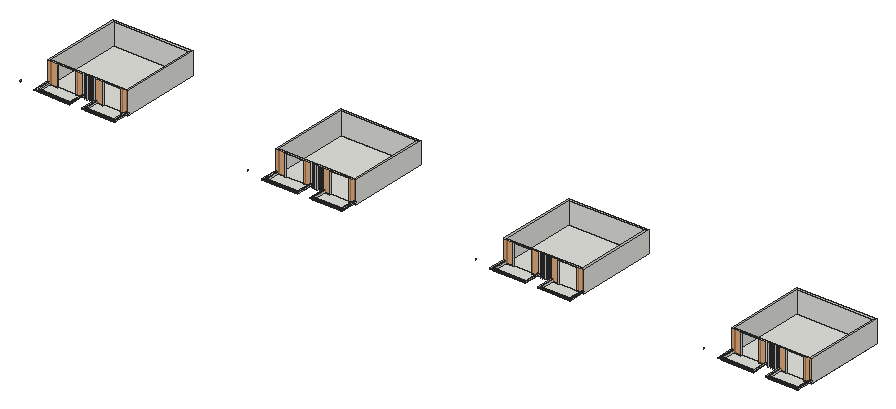
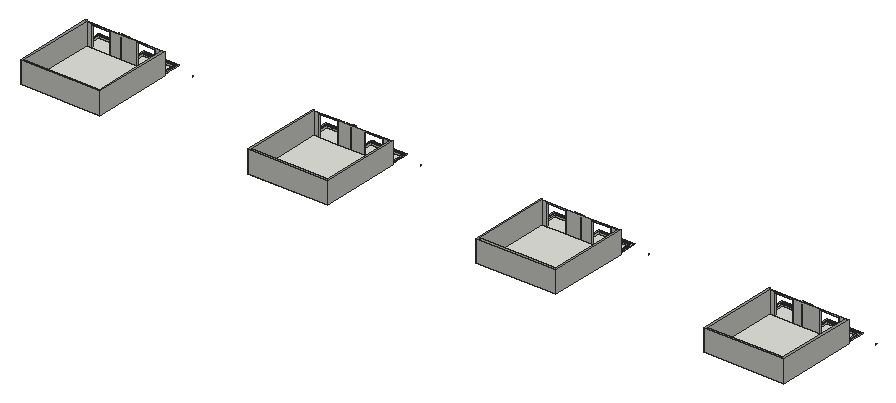
# SketchUp Ruby script. Lengths in inches.
U = 1.inch
M = Sketchup.active_model
def pt(a) = Geom::Point3d.new(a.map { |v| v * U })
def face(e, loops, mat)
  f = e.add_face(loops[0].map { |a| pt(a) })
  loops[1..].each { |l| e.add_face(l.map { |a| pt(a) }).erase! }
  f.material = f.back_material = mat if mat
  f
end
# faces: each face lists its corners as indices into pts; further lists are holes
def faces(e, pts, list, mat = nil) = list.each { |f| face(e, (f[0].is_a?(Array) ? f : [f]).map { |l| l.map { |i| pts[i] } }, mat) }
# xy, xz, yz: faces in a plane at the given z, y or x. An outline is a flat list of corners, or four numbers for a rectangle; further outlines are holes
def ring(l) = l.size == 4 ? [[l[0], l[1]], [l[2], l[1]], [l[2], l[3]], [l[0], l[3]]] : l.each_slice(2).to_a
def flat(e, list, mat, &to3) = list.each { |f| face(e, (f[0].is_a?(Array) ? f : [f]).map { |l| ring(l).map { |u, v| to3.(u, v) } }, mat) }
def xy(e, z, list, mat = nil) = flat(e, list, mat) { |x, y| [x, y, z] }
def xz(e, y, list, mat = nil) = flat(e, list, mat) { |x, z| [x, y, z] }
def yz(e, x, list, mat = nil) = flat(e, list, mat) { |y, z| [x, y, z] }
def lines(e, pts, list) = list.each { |a, b| e.add_line(pt(pts[a]), pt(pts[b])) }
# prism: a flat outline (further loops are holes) pulled along v
def prism(e, loops, v, mat = nil)
  f = face(e, loops, mat); d = Geom::Vector3d.new(v.map { |x| x * U })
  f.pushpull(f.normal.samedirection?(d) ? d.length : -d.length)
end
def box(e, o, s, mat = nil) = prism(e, [[o, [o[0] + s[0], o[1], o[2]], [o[0] + s[0], o[1] + s[1], o[2]], [o[0], o[1] + s[1], o[2]]]], [0, 0, s[2]], mat)
def at(x, y, z, deg = 0) = Geom::Transformation.translation(pt([x, y, z])) * Geom::Transformation.rotation(ORIGIN, Z_AXIS, deg.degrees)
def axes(o, x, y, z) = Geom::Transformation.new([*x, 0, *y, 0, *z, 0, *pt(o).to_a, 1])
def part(name) = M.definitions.add(name)
# library, detail: a bought-in or finely detailed component or shape, given as its bounding box
def library(name, o, s) = part(name).tap { |d| box(d.entities, o, s) }
def detail(e, o, s) = box(e.add_group.entities, o, s)
def put(e, d, t, mat = nil) = e.add_instance(d, t).tap { |i| i.material = mat if mat }
def group(e, t, mat = nil) = e.add_group.tap { |g| g.transformation = t; g.material = mat if mat }.entities
root = M.entities
M.materials.add("[0043_SaddleBrown]4").color = [124, 123, 122]
M.materials.add("[Granite Light Gray]").color = [149, 148, 144]
M.materials.add("[Wood Floor]").color = [224, 152, 88]
M.materials["[Wood Floor]"].alpha = 0.68
xy(root,652.4375,[[563.08,570.83,736.65,570.83,736.65,651.03,703.26,651.03,703.26,657.03,602.01,657.03,602.01,651.03,563.08,651.03],[820.97,570.83,978.86,570.83,978.86,651.03,951.01,651.03,951.01,657.03,849.76,657.03,849.76,651.03,820.97,651.03],[1813.71,570.83,1987.28,570.83,1987.28,651.03,1953.89,651.03,1953.89,657.03,1852.64,657.03,1852.64,651.03,1813.71,651.03],[2071.59,570.83,2229.49,570.83,2229.49,651.03,2201.63,651.03,2201.63,657.03,2100.38,657.03,2100.38,651.03,2071.59,651.03],[3064.33,570.83,3237.9,570.83,3237.9,651.03,3204.51,651.03,3204.51,657.03,3103.26,657.03,3103.26,651.03,3064.33,651.03],
  [3322.22,570.83,3480.11,570.83,3480.11,651.03,3452.26,651.03,3452.26,657.03,3351.01,657.03,3351.01,651.03,3322.22,651.03],[4314.96,570.83,4488.53,570.83,4488.53,651.03,4455.14,651.03,4455.14,657.03,4353.89,657.03,4353.89,651.03,4314.96,651.03],[4572.84,570.83,4730.74,570.83,4730.74,651.03,4702.88,651.03,4702.88,657.03,4601.63,657.03,4601.63,651.03,4572.84,651.03],[551.76,651.03,551.76,1096.5,990.19,1096.5,990.19,651.03,951.01,651.03,951.01,657.03,978.86,657.03,978.86,1085.17,563.08,1085.17,563.08,657.03,602.01,657.03,602.01,651.03],[1802.38,651.03,1802.38,1096.5,2240.81,1096.5,2240.81,651.03,2201.63,651.03,2201.63,657.03,2229.49,657.03,2229.49,1085.17,1813.71,1085.17,1813.71,657.03,1852.64,657.03,1852.64,651.03],
  [3053.01,651.03,3053.01,1096.5,3491.44,1096.5,3491.44,651.03,3452.26,651.03,3452.26,657.03,3480.11,657.03,3480.11,1085.17,3064.33,1085.17,3064.33,657.03,3103.26,657.03,3103.26,651.03],[4303.63,651.03,4303.63,1096.5,4742.06,1096.5,4742.06,651.03,4702.88,651.03,4702.88,657.03,4730.74,657.03,4730.74,1085.17,4314.96,1085.17,4314.96,657.03,4353.89,657.03,4353.89,651.03],[563.08,657.03,978.86,1085.17],[1813.71,657.03,2229.49,1085.17],[3064.33,657.03,3480.11,1085.17],
  [4314.96,657.03,4730.74,1085.17]])
xy(root,662.4375,[[549.88,558.125,744.19,559.875],[812.81,558.125,990.19,559.875],[990.19,558.125,991.94,651.03],[1800.51,558.125,1994.82,559.875],[2063.43,558.125,2240.81,559.875],
  [2240.81,558.125,2242.56,651.03],[3051.13,558.125,3245.44,559.875],[3314.06,558.125,3491.44,559.875],[3491.44,558.125,3493.19,651.03],[4301.76,558.125,4496.07,559.875],
  [4564.68,558.125,4742.06,559.875],[4742.06,558.125,4743.81,651.03],[549.88,559.875,551.76,640.11],[551.76,559.875,551.76,651.03,563.08,651.03,563.08,570.83,736.65,570.83,736.65,651.03,742.44,651.03,742.44,559.875],[742.44,559.875,744.19,647.91],
  [812.81,559.875,812.81,648.85,814.68,648.85,814.68,651.03,814.89,651.03,814.89,559.875],[814.89,559.875,814.89,651.03,820.97,651.03,820.97,570.83,978.86,570.83,978.86,651.03,990.19,651.03,990.19,559.875],[1800.51,559.875,1802.38,640.11],[1802.38,559.875,1802.38,651.03,1813.71,651.03,1813.71,570.83,1987.28,570.83,1987.28,651.03,1993.07,651.03,1993.07,559.875],[1993.07,559.875,1994.82,647.91],
  [2063.43,559.875,2063.43,648.85,2065.31,648.85,2065.31,651.03,2065.52,651.03,2065.52,559.875],[2065.52,559.875,2065.52,651.03,2071.59,651.03,2071.59,570.83,2229.49,570.83,2229.49,651.03,2240.81,651.03,2240.81,559.875],[3051.13,559.875,3053.01,640.11],[3053.01,559.875,3053.01,651.03,3064.33,651.03,3064.33,570.83,3237.9,570.83,3237.9,651.03,3243.69,651.03,3243.69,559.875],[3243.69,559.875,3245.44,647.91],
  [3314.06,559.875,3314.06,648.85,3315.93,648.85,3315.93,651.03,3316.14,651.03,3316.14,559.875],[3316.14,559.875,3316.14,651.03,3322.22,651.03,3322.22,570.83,3480.11,570.83,3480.11,651.03,3491.44,651.03,3491.44,559.875],[4301.76,559.875,4303.63,640.11],[4303.63,559.875,4303.63,651.03,4314.96,651.03,4314.96,570.83,4488.53,570.83,4488.53,651.03,4494.32,651.03,4494.32,559.875],[4494.32,559.875,4496.07,647.91],
  [4564.68,559.875,4564.68,648.85,4566.56,648.85,4566.56,651.03,4566.77,651.03,4566.77,559.875],[4566.77,559.875,4566.77,651.03,4572.84,651.03,4572.84,570.83,4730.74,570.83,4730.74,651.03,4742.06,651.03,4742.06,559.875]])
xz(root,558.125,[[549.88,662.4375,744.19,665.9375],[812.81,662.4375,991.94,665.9375],[1800.51,662.4375,1994.82,665.9375],[2063.43,662.4375,2242.56,665.9375],[3051.13,662.4375,3245.44,665.9375],
  [3314.06,662.4375,3493.19,665.9375],[4301.76,662.4375,4496.07,665.9375],[4564.68,662.4375,4743.81,665.9375]],"[Granite Light Gray]")
xz(root,570.83,[[563.08,652.4375,736.65,662.4375],[820.97,652.4375,978.86,662.4375],[1813.71,652.4375,1987.28,662.4375],[2071.59,652.4375,2229.49,662.4375],[3064.33,652.4375,3237.9,662.4375],
  [3322.22,652.4375,3480.11,662.4375],[4314.96,652.4375,4488.53,662.4375],[4572.84,652.4375,4730.74,662.4375],[563.08,662.4375,736.65,665.9375],[820.97,662.4375,978.86,665.9375],
  [1813.71,662.4375,1987.28,665.9375],[2071.59,662.4375,2229.49,665.9375],[3064.33,662.4375,3237.9,665.9375],[3322.22,662.4375,3480.11,665.9375],[4314.96,662.4375,4488.53,665.9375],
  [4572.84,662.4375,4730.74,665.9375]])
xz(root,589.17,[[449.07,657.09,449.07,663.29,448.85,662.79,448.66,662.27,448.52,661.76,448.42,661.24,448.35,660.72,448.33,660.19,448.35,659.67,448.42,659.14,448.52,658.625,448.66,658.11,448.85,657.6],[1699.7,657.09,1699.7,663.29,1699.47,662.79,1699.29,662.27,1699.14,661.76,1699.04,661.24,1698.98,660.72,1698.96,660.19,1698.98,659.67,1699.04,659.14,1699.14,658.625,1699.29,658.11,1699.47,657.6],[2950.32,657.09,2950.32,663.29,2950.1,662.79,2949.91,662.27,2949.77,661.76,2949.67,661.24,2949.6,660.72,2949.58,660.19,2949.6,659.67,2949.67,659.14,2949.77,658.625,2949.91,658.11,2950.1,657.6],[4200.95,657.09,4200.95,663.29,4200.72,662.79,4200.54,662.27,4200.39,661.76,4200.29,661.24,4200.23,660.72,4200.21,660.19,4200.23,659.67,4200.29,659.14,4200.39,658.625,4200.54,658.11,4200.72,657.6]],"[0043_SaddleBrown]4")
xz(root,640.11,[[549.88,662.4375,551.76,665.9375],[1800.51,662.4375,1802.38,665.9375],[3051.13,662.4375,3053.01,665.9375],[4301.76,662.4375,4303.63,665.9375]])
xz(root,647.91,[[742.44,662.4375,744.19,665.9375],[1993.07,662.4375,1994.82,665.9375],[3243.69,662.4375,3245.44,665.9375],[4494.32,662.4375,4496.07,665.9375]])
xz(root,648.85,[[812.81,662.4375,814.68,665.9375],[2063.43,662.4375,2065.31,665.9375],[3314.06,662.4375,3315.93,665.9375],[4564.68,662.4375,4566.56,665.9375]])
xz(root,651.03,[[551.76,652.4375,563.08,662.4375],[978.86,652.4375,990.19,662.4375],[1802.38,652.4375,1813.71,662.4375],[2229.49,652.4375,2240.81,662.4375],[3053.01,652.4375,3064.33,662.4375],
  [3480.11,652.4375,3491.44,662.4375],[4303.63,652.4375,4314.96,662.4375],[4730.74,652.4375,4742.06,662.4375],[551.76,662.4375,563.08,665.9375],[736.65,662.4375,742.44,665.9375],
  [814.68,662.4375,820.97,665.9375],[978.86,662.4375,990.19,665.9375],[990.19,662.4375,991.94,665.9375],[1802.38,662.4375,1813.71,665.9375],[1987.28,662.4375,1993.07,665.9375],
  [2065.31,662.4375,2071.59,665.9375],[2229.49,662.4375,2240.81,665.9375],[2240.81,662.4375,2242.56,665.9375],[3053.01,662.4375,3064.33,665.9375],[3237.9,662.4375,3243.69,665.9375],
  [3315.93,662.4375,3322.22,665.9375],[3480.11,662.4375,3491.44,665.9375],[3491.44,662.4375,3493.19,665.9375],[4303.63,662.4375,4314.96,665.9375],[4488.53,662.4375,4494.32,665.9375],
  [4566.56,662.4375,4572.84,665.9375],[4730.74,662.4375,4742.06,665.9375],[4742.06,662.4375,4743.81,665.9375]])
xz(root,651.03,[[563.08,652.4375,602.01,652.4375,602.01,766.875,703.26,766.875,703.26,652.4375,736.65,652.4375,736.65,665.9375,742.44,665.9375,742.44,771.4375,551.76,771.4375,551.76,665.9375,563.08,665.9375],[820.97,652.4375,849.76,652.4375,849.76,766.875,951.01,766.875,951.01,652.4375,978.86,652.4375,978.86,665.9375,990.19,665.9375,990.19,772.4375,978.86,772.4375,978.86,776.0625,977.59,776.0625,977.59,771.4375,814.89,771.4375,814.89,665.9375,820.97,665.9375],[1813.71,652.4375,1852.64,652.4375,1852.64,766.875,1953.89,766.875,1953.89,652.4375,1987.28,652.4375,1987.28,665.9375,1993.07,665.9375,1993.07,771.4375,1802.38,771.4375,1802.38,665.9375,1813.71,665.9375],[2071.59,652.4375,2100.38,652.4375,2100.38,766.875,2201.63,766.875,2201.63,652.4375,2229.49,652.4375,2229.49,665.9375,2240.81,665.9375,2240.81,772.4375,2229.49,772.4375,2229.49,776.0625,2228.22,776.0625,2228.22,771.4375,2065.52,771.4375,2065.52,665.9375,2071.59,665.9375],[3064.33,652.4375,3103.26,652.4375,3103.26,766.875,3204.51,766.875,3204.51,652.4375,3237.9,652.4375,3237.9,665.9375,3243.69,665.9375,3243.69,771.4375,3053.01,771.4375,3053.01,665.9375,3064.33,665.9375],
  [3322.22,652.4375,3351.01,652.4375,3351.01,766.875,3452.26,766.875,3452.26,652.4375,3480.11,652.4375,3480.11,665.9375,3491.44,665.9375,3491.44,772.4375,3480.11,772.4375,3480.11,776.0625,3478.84,776.0625,3478.84,771.4375,3316.14,771.4375,3316.14,665.9375,3322.22,665.9375],[4314.96,652.4375,4353.89,652.4375,4353.89,766.875,4455.14,766.875,4455.14,652.4375,4488.53,652.4375,4488.53,665.9375,4494.32,665.9375,4494.32,771.4375,4303.63,771.4375,4303.63,665.9375,4314.96,665.9375],[4572.84,652.4375,4601.63,652.4375,4601.63,766.875,4702.88,766.875,4702.88,652.4375,4730.74,652.4375,4730.74,665.9375,4742.06,665.9375,4742.06,772.4375,4730.74,772.4375,4730.74,776.0625,4729.47,776.0625,4729.47,771.4375,4566.77,771.4375,4566.77,665.9375,4572.84,665.9375]],"[Wood Floor]")
xz(root,657.03,[[563.08,652.4375,563.08,772.4375,978.86,772.4375,978.86,652.4375,951.01,652.4375,951.01,766.875,849.76,766.875,849.76,652.4375,703.26,652.4375,703.26,766.875,602.01,766.875,602.01,652.4375],[1813.71,652.4375,1813.71,772.4375,2229.49,772.4375,2229.49,652.4375,2201.63,652.4375,2201.63,766.875,2100.38,766.875,2100.38,652.4375,1953.89,652.4375,1953.89,766.875,1852.64,766.875,1852.64,652.4375],[3064.33,652.4375,3064.33,772.4375,3480.11,772.4375,3480.11,652.4375,3452.26,652.4375,3452.26,766.875,3351.01,766.875,3351.01,652.4375,3204.51,652.4375,3204.51,766.875,3103.26,766.875,3103.26,652.4375],[4314.96,652.4375,4314.96,772.4375,4730.74,772.4375,4730.74,652.4375,4702.88,652.4375,4702.88,766.875,4601.63,766.875,4601.63,652.4375,4455.14,652.4375,4455.14,766.875,4353.89,766.875,4353.89,652.4375]])
xz(root,1085.17,[[563.08,652.4375,978.86,772.4375],[1813.71,652.4375,2229.49,772.4375],[3064.33,652.4375,3480.11,772.4375],[4314.96,652.4375,4730.74,772.4375]])
xz(root,1096.5,[[551.76,652.4375,990.19,772.4375],[1802.38,652.4375,2240.81,772.4375],[3053.01,652.4375,3491.44,772.4375],[4303.63,652.4375,4742.06,772.4375]])
yz(root,549.88,[[558.125,662.4375,640.11,665.9375]])
yz(root,551.76,[[651.03,652.4375,1096.5,772.4375],[640.11,662.4375,651.03,665.9375]])
yz(root,563.08,[[570.83,652.4375,651.03,662.4375],[657.03,652.4375,1085.17,772.4375],[570.83,662.4375,651.03,665.9375]])
yz(root,602.01,[[651.03,652.4375,657.03,766.875]])
yz(root,703.26,[[651.03,652.4375,657.03,766.875]])
yz(root,736.65,[[570.83,652.4375,651.03,662.4375],[570.83,662.4375,651.03,665.9375]])
yz(root,742.44,[[647.91,662.4375,651.03,665.9375]])
yz(root,744.19,[[558.125,662.4375,647.91,665.9375]])
yz(root,755.44,[[647.91,652.4375,651.03,771.4375]])
yz(root,768.19,[[648.85,652.4375,651.03,771.4375]])
yz(root,780.32,[[648.85,652.4375,651.03,771.4375]])
yz(root,792.69,[[648.85,652.4375,651.03,771.4375]])
yz(root,805.57,[[648.85,652.4375,651.03,771.4375]])
yz(root,812.81,[[558.125,662.4375,648.85,665.9375]])
yz(root,814.68,[[648.85,662.4375,651.03,665.9375]])
yz(root,820.97,[[570.83,652.4375,651.03,662.4375],[570.83,662.4375,651.03,665.9375]])
yz(root,849.76,[[651.03,652.4375,657.03,766.875]])
yz(root,951.01,[[651.03,652.4375,657.03,766.875]])
yz(root,978.86,[[570.83,652.4375,651.03,662.4375],[657.03,652.4375,1085.17,772.4375],[570.83,662.4375,651.03,665.9375]])
yz(root,990.19,[[651.03,652.4375,1096.5,772.4375]])
yz(root,991.94,[[558.125,662.4375,651.03,665.9375]])
yz(root,1800.51,[[558.125,662.4375,640.11,665.9375]])
yz(root,1802.38,[[651.03,652.4375,1096.5,772.4375],[640.11,662.4375,651.03,665.9375]])
yz(root,1813.71,[[570.83,652.4375,651.03,662.4375],[657.03,652.4375,1085.17,772.4375],[570.83,662.4375,651.03,665.9375]])
yz(root,1852.64,[[651.03,652.4375,657.03,766.875]])
yz(root,1953.89,[[651.03,652.4375,657.03,766.875]])
yz(root,1987.28,[[570.83,652.4375,651.03,662.4375],[570.83,662.4375,651.03,665.9375]])
yz(root,1993.07,[[647.91,662.4375,651.03,665.9375]])
yz(root,1994.82,[[558.125,662.4375,647.91,665.9375]])
yz(root,2006.07,[[647.91,652.4375,651.03,771.4375]])
yz(root,2018.82,[[648.85,652.4375,651.03,771.4375]])
yz(root,2030.94,[[648.85,652.4375,651.03,771.4375]])
yz(root,2043.32,[[648.85,652.4375,651.03,771.4375]])
yz(root,2056.19,[[648.85,652.4375,651.03,771.4375]])
yz(root,2063.43,[[558.125,662.4375,648.85,665.9375]])
yz(root,2065.31,[[648.85,662.4375,651.03,665.9375]])
yz(root,2071.59,[[570.83,652.4375,651.03,662.4375],[570.83,662.4375,651.03,665.9375]])
yz(root,2100.38,[[651.03,652.4375,657.03,766.875]])
yz(root,2201.63,[[651.03,652.4375,657.03,766.875]])
yz(root,2229.49,[[570.83,652.4375,651.03,662.4375],[657.03,652.4375,1085.17,772.4375],[570.83,662.4375,651.03,665.9375]])
yz(root,2240.81,[[651.03,652.4375,1096.5,772.4375]])
yz(root,2242.56,[[558.125,662.4375,651.03,665.9375]])
yz(root,3051.13,[[558.125,662.4375,640.11,665.9375]])
yz(root,3053.01,[[651.03,652.4375,1096.5,772.4375],[640.11,662.4375,651.03,665.9375]])
yz(root,3064.33,[[570.83,652.4375,651.03,662.4375],[657.03,652.4375,1085.17,772.4375],[570.83,662.4375,651.03,665.9375]])
yz(root,3103.26,[[651.03,652.4375,657.03,766.875]])
yz(root,3204.51,[[651.03,652.4375,657.03,766.875]])
yz(root,3237.9,[[570.83,652.4375,651.03,662.4375],[570.83,662.4375,651.03,665.9375]])
yz(root,3243.69,[[647.91,662.4375,651.03,665.9375]])
yz(root,3245.44,[[558.125,662.4375,647.91,665.9375]])
yz(root,3256.69,[[647.91,652.4375,651.03,771.4375]])
yz(root,3269.44,[[648.85,652.4375,651.03,771.4375]])
yz(root,3281.57,[[648.85,652.4375,651.03,771.4375]])
yz(root,3293.94,[[648.85,652.4375,651.03,771.4375]])
yz(root,3306.82,[[648.85,652.4375,651.03,771.4375]])
yz(root,3314.06,[[558.125,662.4375,648.85,665.9375]])
yz(root,3315.93,[[648.85,662.4375,651.03,665.9375]])
yz(root,3322.22,[[570.83,652.4375,651.03,662.4375],[570.83,662.4375,651.03,665.9375]])
yz(root,3351.01,[[651.03,652.4375,657.03,766.875]])
yz(root,3452.26,[[651.03,652.4375,657.03,766.875]])
yz(root,3480.11,[[570.83,652.4375,651.03,662.4375],[657.03,652.4375,1085.17,772.4375],[570.83,662.4375,651.03,665.9375]])
yz(root,3491.44,[[651.03,652.4375,1096.5,772.4375]])
yz(root,3493.19,[[558.125,662.4375,651.03,665.9375]])
yz(root,4301.76,[[558.125,662.4375,640.11,665.9375]])
yz(root,4303.63,[[651.03,652.4375,1096.5,772.4375],[640.11,662.4375,651.03,665.9375]])
yz(root,4314.96,[[570.83,652.4375,651.03,662.4375],[657.03,652.4375,1085.17,772.4375],[570.83,662.4375,651.03,665.9375]])
yz(root,4353.89,[[651.03,652.4375,657.03,766.875]])
yz(root,4455.14,[[651.03,652.4375,657.03,766.875]])
yz(root,4488.53,[[570.83,652.4375,651.03,662.4375],[570.83,662.4375,651.03,665.9375]])
yz(root,4494.32,[[647.91,662.4375,651.03,665.9375]])
yz(root,4496.07,[[558.125,662.4375,647.91,665.9375]])
yz(root,4507.32,[[647.91,652.4375,651.03,771.4375]])
yz(root,4520.07,[[648.85,652.4375,651.03,771.4375]])
yz(root,4532.19,[[648.85,652.4375,651.03,771.4375]])
yz(root,4544.57,[[648.85,652.4375,651.03,771.4375]])
yz(root,4557.44,[[648.85,652.4375,651.03,771.4375]])
yz(root,4564.68,[[558.125,662.4375,648.85,665.9375]])
yz(root,4566.56,[[648.85,662.4375,651.03,665.9375]])
yz(root,4572.84,[[570.83,652.4375,651.03,662.4375],[570.83,662.4375,651.03,665.9375]])
yz(root,4601.63,[[651.03,652.4375,657.03,766.875]])
yz(root,4702.88,[[651.03,652.4375,657.03,766.875]])
yz(root,4730.74,[[570.83,652.4375,651.03,662.4375],[657.03,652.4375,1085.17,772.4375],[570.83,662.4375,651.03,665.9375]])
yz(root,4742.06,[[651.03,652.4375,1096.5,772.4375]])
yz(root,4743.81,[[558.125,662.4375,651.03,665.9375]])
